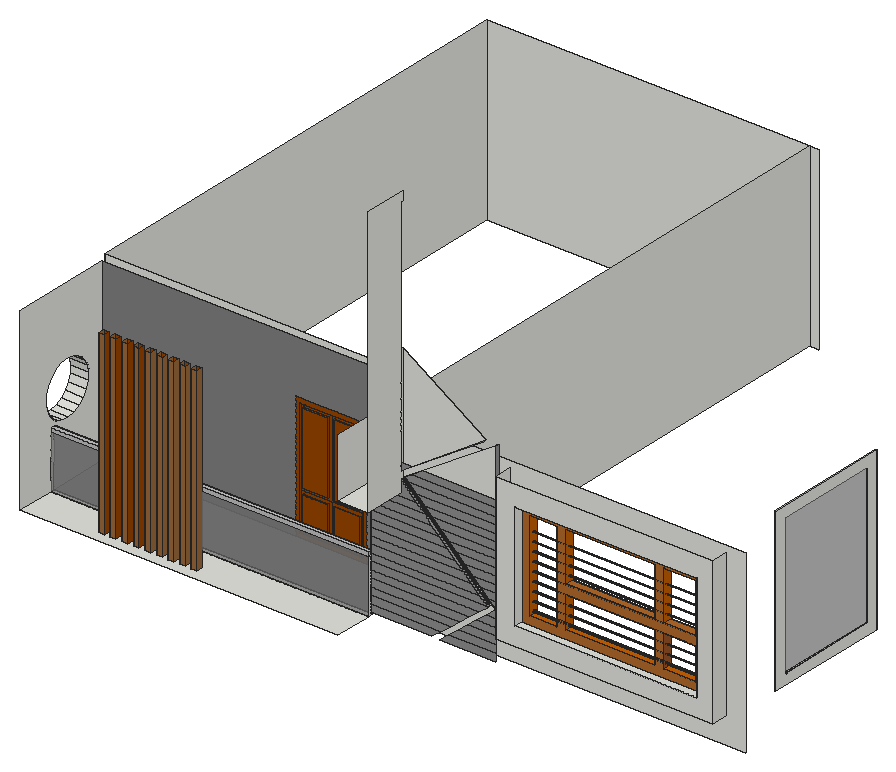
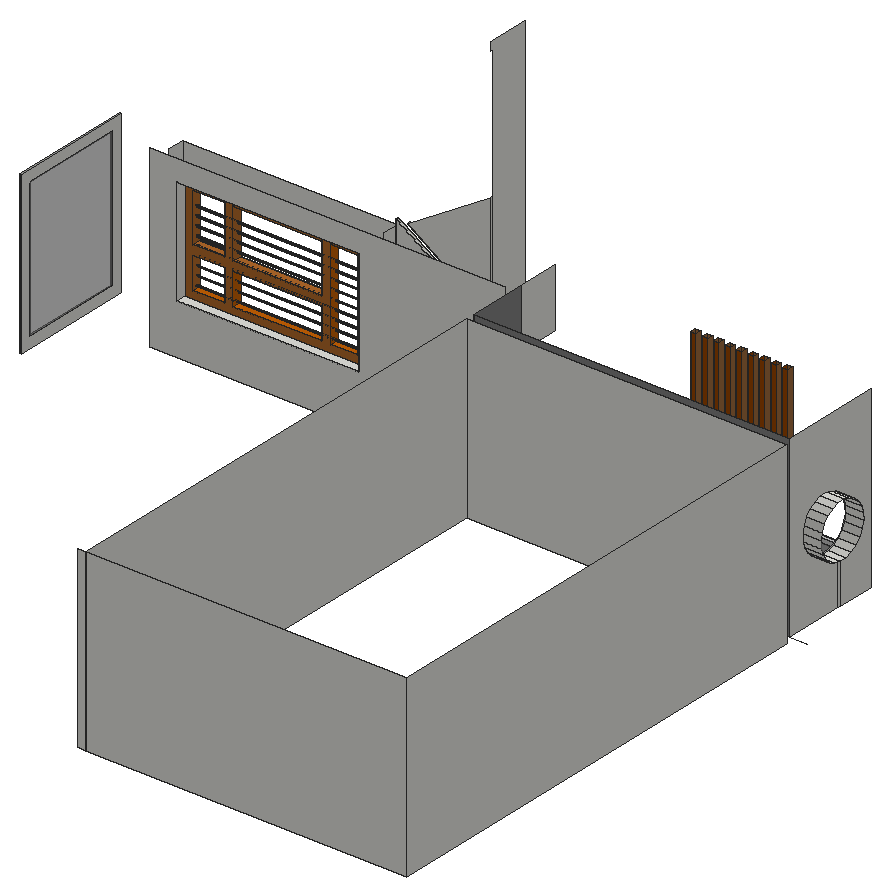
# SketchUp Ruby script. Lengths in inches.
U = 1.inch
M = Sketchup.active_model
def pt(a) = Geom::Point3d.new(a.map { |v| v * U })
def face(e, loops, mat)
  f = e.add_face(loops[0].map { |a| pt(a) })
  loops[1..].each { |l| e.add_face(l.map { |a| pt(a) }).erase! }
  f.material = f.back_material = mat if mat
  f
end
# faces: each face lists its corners as indices into pts; further lists are holes
def faces(e, pts, list, mat = nil) = list.each { |f| face(e, (f[0].is_a?(Array) ? f : [f]).map { |l| l.map { |i| pts[i] } }, mat) }
# xy, xz, yz: faces in a plane at the given z, y or x. An outline is a flat list of corners, or four numbers for a rectangle; further outlines are holes
def ring(l) = l.size == 4 ? [[l[0], l[1]], [l[2], l[1]], [l[2], l[3]], [l[0], l[3]]] : l.each_slice(2).to_a
def flat(e, list, mat, &to3) = list.each { |f| face(e, (f[0].is_a?(Array) ? f : [f]).map { |l| ring(l).map { |u, v| to3.(u, v) } }, mat) }
def xy(e, z, list, mat = nil) = flat(e, list, mat) { |x, y| [x, y, z] }
def xz(e, y, list, mat = nil) = flat(e, list, mat) { |x, z| [x, y, z] }
def yz(e, x, list, mat = nil) = flat(e, list, mat) { |y, z| [x, y, z] }
def lines(e, pts, list) = list.each { |a, b| e.add_line(pt(pts[a]), pt(pts[b])) }
# prism: a flat outline (further loops are holes) pulled along v
def prism(e, loops, v, mat = nil)
  f = face(e, loops, mat); d = Geom::Vector3d.new(v.map { |x| x * U })
  f.pushpull(f.normal.samedirection?(d) ? d.length : -d.length)
end
def box(e, o, s, mat = nil) = prism(e, [[o, [o[0] + s[0], o[1], o[2]], [o[0] + s[0], o[1] + s[1], o[2]], [o[0], o[1] + s[1], o[2]]]], [0, 0, s[2]], mat)
def at(x, y, z, deg = 0) = Geom::Transformation.translation(pt([x, y, z])) * Geom::Transformation.rotation(ORIGIN, Z_AXIS, deg.degrees)
def axes(o, x, y, z) = Geom::Transformation.new([*x, 0, *y, 0, *z, 0, *pt(o).to_a, 1])
def part(name) = M.definitions.add(name)
# library, detail: a bought-in or finely detailed component or shape, given as its bounding box
def library(name, o, s) = part(name).tap { |d| box(d.entities, o, s) }
def detail(e, o, s) = box(e.add_group.entities, o, s)
def put(e, d, t, mat = nil) = e.add_instance(d, t).tap { |i| i.material = mat if mat }
def group(e, t, mat = nil) = e.add_group.tap { |g| g.transformation = t; g.material = mat if mat }.entities
root = M.entities
M.materials.add("[0132_LightGray]").color = [169, 169, 169]
M.materials.add("[0133_Gray]").color = [128, 128, 128]
M.materials.add("[Color M04]").color = [142, 142, 142]
M.materials.add("[Metal Corrugated Shiny]").color = [193, 193, 193]
M.materials.add("[Stone Vein Gray]").color = [166, 165, 165]
M.materials.add("[Translucent Glass Gray]").color = [128, 128, 128]
M.materials["[Translucent Glass Gray]"].alpha = 0.68
M.materials.add("[Wood Bamboo]").color = [195, 96, 5]
M.materials.add("[Wood Bamboo]1").color = [177, 105, 43]
M.materials.add("[Wood Cherry Original]").color = [152, 68, 0]
M.materials.add("[Wood Cherry Original]1").color = [152, 86, 42]
M.materials.add("[Wood Floor]").color = [155, 105, 61]
xy(root,218,[[[28.03,15.6875,241.25,41],[74.77,23.01,78.7,26.95],[82.52,23.01,86.45,26.95],[90.27,23.01,94.2,26.95],[98.02,23.01,101.95,26.95],[105.77,23.01,109.7,26.95],[113.52,23.01,117.45,26.95],[121.27,23.01,125.2,26.95],[129.02,23.01,132.95,26.95],[136.77,23.01,140.7,26.95]],[28.03,41,241.25,44]])
xy(root,218,[[28.03,44,241.25,84.25]],"[Stone Vein Gray]")
xy(root,218,[[74.77,23.01,78.7,26.95],[82.52,23.01,86.45,26.95],[90.27,23.01,94.2,26.95],[98.02,23.01,101.95,26.95],[105.77,23.01,109.7,26.95],
  [113.52,23.01,117.45,26.95],[121.27,23.01,125.2,26.95],[129.02,23.01,132.95,26.95],[136.77,23.01,140.7,26.95]],"[Wood Cherry Original]")
xy(root,220.79,[[160.66,84.25,203.09,84.75]],"[Wood Cherry Original]")
xy(root,222.79,[[162.66,83.75,179.875,84.75]])
xy(root,222.82,[[183.91,83.75,201.05,84.75]])
xy(root,239.94,[[333.13,33.25,478.31,44.6875]])
xy(root,244.7,[[183.91,83.75,201.05,84.75]],"[Wood Cherry Original]")
xy(root,244.74,[[162.66,83.75,179.875,84.75]],"[Wood Cherry Original]")
xy(root,248.74,[[162.66,83.75,179.875,84.75],[183.875,83.75,201.09,84.75]])
xy(root,252.35,[[345.84,33.25,468.09,38.65],[345.84,44.67,468.09,50.6875]])
xy(root,253,[[495.875,63.375,496.875,147.375]])
xy(root,254,[[28.03,41,241.25,44]],"[Metal Corrugated Shiny]")
xy(root,256.625,[[28.03,41,241.25,44]],"[Metal Corrugated Shiny]")
xy(root,257.74,[[351.24,38.65,369.24,44.67],[375.24,38.65,435.1,44.67],[441.1,38.65,462.7,44.67]],"[Wood Bamboo]")
xy(root,260,[[495.875,70.375,496.875,140.375]])
xy(root,279.34,[[375.24,38.65,435.1,44.67],[441.1,38.65,462.7,44.67]])
xy(root,285.34,[[375.24,38.65,435.1,44.67],[441.1,38.65,462.7,44.67]],"[Wood Bamboo]1")
xy(root,297.21,[[162.66,83.75,179.875,84.75],[183.875,83.75,201.09,84.75]],"[Wood Cherry Original]")
xy(root,298.5,[[241.25,15.6875,261.37,42.75],[241.25,42.75,261.37,44.4375],[241.25,44.4375,261.37,44.6875]])
xy(root,299.21,[[160.66,84.25,203.09,84.75]])
xz(root,23.01,[[74.77,218,78.7,338],[82.52,218,86.45,338],[90.27,218,94.2,338],[98.02,218,101.95,338],[105.77,218,109.7,338],
  [113.52,218,117.45,338],[121.27,218,125.2,338],[129.02,218,132.95,338],[136.77,218,140.7,338]],"[Wood Floor]")
xz(root,26.95,[[74.77,218,78.7,338],[82.52,218,86.45,338],[90.27,218,94.2,338],[98.02,218,101.95,338],[105.77,218,109.7,338],
  [113.52,218,117.45,338],[121.27,218,125.2,338],[129.02,218,132.95,338],[136.77,218,140.7,338]],"[Wood Cherry Original]")
xz(root,33.25,[[[333.13,239.94,478.31,337.75],[345.84,252.35,468.09,323.97]]])
xz(root,38.65,[[[345.84,252.35,468.09,323.97],[375.24,257.74,375.24,279.34,435.1,279.34,435.1,257.74,441.1,257.74,441.1,279.34,462.7,279.34,462.7,285.34,441.1,285.34,441.1,318.58,462.7,318.58,462.7,257.74],[375.24,285.34,435.1,318.58],[351.24,257.74,369.24,318.58]]],"[Wood Bamboo]1")
xz(root,41,[[28.03,254,241.25,256.625]],"[Metal Corrugated Shiny]")
xz(root,41,[[28.03,218,241.25,254]],"[Translucent Glass Gray]")
xz(root,42.75,[[325.43,250.42,325.49,250.42,325.49,250.46]])
xz(root,42.75,[[241.25,219.67,282.3,219.67,288.6,224.79,241.25,224.79],[287.88,219.67,325.49,219.67,325.49,224.79,294.14,224.79],[241.25,224.79,288.6,224.79,294.9,229.92,241.25,229.92],[294.14,224.79,325.49,224.79,325.49,229.92,300.4,229.92],[241.25,229.92,294.9,229.92,301.2,235.04,241.25,235.04],
  [300.4,229.92,325.49,229.92,325.49,235.04,306.66,235.04],[241.25,235.04,301.2,235.04,307.51,240.17,241.25,240.17],[306.66,235.04,325.49,235.04,325.49,240.17,312.92,240.17],[241.25,240.17,307.51,240.17,313.81,245.29,241.25,245.29],[312.92,240.17,325.49,240.17,325.49,245.29,319.17,245.29],
  [241.25,245.29,313.81,245.29,319.9,250.25,319.73,250.42,241.25,250.42],[319.17,245.29,325.49,245.29,325.49,250.42,325.43,250.42],[241.25,250.42,319.73,250.42,314.4375,255.54,241.25,255.54],[325.49,250.46,325.49,255.54,320.17,255.54],[241.25,255.54,314.4375,255.54,309.15,260.67,241.25,260.67],
  [320.17,255.54,325.49,255.54,325.49,260.67,314.8125,260.67],[241.25,260.67,309.15,260.67,303.86,265.79,241.25,265.79],[314.8125,260.67,325.49,260.67,325.49,265.79,309.45,265.79],[241.25,265.79,303.86,265.79,298.57,270.92,241.25,270.92],[309.45,265.79,325.49,265.79,325.49,270.92,304.09,270.92],
  [241.25,270.92,298.57,270.92,293.28,276.04,241.25,276.04],[304.09,270.92,325.49,270.92,325.49,276.04,298.73,276.04],[241.25,276.04,293.28,276.04,287.99,281.17,241.25,281.17],[298.73,276.04,325.49,276.04,325.49,281.17,293.375,281.17],[241.25,281.17,287.99,281.17,282.7,286.29,241.25,286.29],
  [293.375,281.17,325.49,281.17,325.49,286.29,288.01,286.29],[241.25,286.29,282.7,286.29,277.41,291.42,241.25,291.42],[288.01,286.29,325.49,286.29,325.49,291.42,282.65,291.42],[241.25,291.42,277.41,291.42,272.125,296.54,241.25,296.54],[282.65,291.42,325.49,291.42,325.49,296.54,277.3,296.54],
  [241.25,296.54,272.125,296.54,261.37,306.96,261.37,298.5,241.25,298.5],[277.3,296.54,325.49,296.54,325.49,301.67,271.9375,301.67],[271.9375,301.67,325.49,301.67,325.49,306.79,266.58,306.79],[266.58,306.79,325.49,306.79,325.49,311.92,268.9,311.92,264.35,308.92],[261.37,311.77,269.28,317.04,261.37,317.04],
  [268.9,311.92,325.49,311.92,325.49,317.04,276.6875,317.04]],"[Color M04]")
xz(root,44,[[28.03,254,241.25,256.625]],"[Metal Corrugated Shiny]")
xz(root,44,[[28.03,218,241.25,254]],"[Translucent Glass Gray]")
xz(root,44.67,[[[345.84,252.35,468.09,323.97],[375.24,285.34,435.1,318.58],[375.24,257.74,435.1,279.34],[351.24,257.74,369.24,318.58],[441.1,285.34,462.7,318.58],[441.1,257.74,462.7,279.34]]],"[Wood Bamboo]1")
xz(root,44.6875,[[325.49,250.46,264.35,308.92,325.49,349.15],[261.37,311.77,261.37,384.6,317.38,349.1]])
xz(root,50.6875,[[[247.25,218,486.875,338],[345.84,252.35,468.09,323.97]]])
xz(root,63.375,[[495.875,253,496.875,361]])
xz(root,70.375,[[495.875,260,496.875,354]])
xz(root,83.75,[[162.66,222.79,179.875,244.74],[183.91,222.82,201.05,244.7],[162.66,248.74,179.875,297.21],[183.875,248.74,201.09,297.21]],"[Wood Cherry Original]")
xz(root,84.25,[[28.03,218,157.875,218,157.875,302,205.875,302,205.875,218,241.25,218,241.25,338,28.03,338]],"[0133_Gray]")
xz(root,84.25,[[[157.875,218,205.875,302],[160.66,220.79,203.09,299.21]]],"[Wood Cherry Original]")
xz(root,84.75,[[[160.66,220.79,181.875,246.74],[162.66,222.79,179.875,244.74]],[[181.875,220.79,203.09,246.74],[183.91,222.82,201.05,244.7]],[[160.66,246.74,181.875,299.21],[162.66,248.74,179.875,297.21]],[[181.875,246.74,203.09,299.21],[183.875,248.74,201.09,297.21]]],"[Wood Cherry Original]")
xz(root,90.25,[[24.875,218,241.25,338]])
xz(root,140.375,[[495.875,260,496.875,354]])
xz(root,147.375,[[495.875,253,496.875,361]])
xz(root,411,[[24.875,218,241.25,338],[241.25,218,247.25,338]])
yz(root,24.875,[[90.25,218,411,338]])
yz(root,28.03,[[[15.6875,218,41,218,41,256.625,44,256.625,44,218,84.25,218,84.25,338,15.6875,338],[56.56,256.125,51.83,256.36,47.33,257.82,43.36,260.38,40.19,263.89,38.03,268.11,37.04,272.73,37.27,277.46,38.73,281.96,41.3,285.93,44.81,289.11,49.02,291.26,53.64,292.26,58.37,292.02,62.87,290.57,66.85,288,70.02,284.49,72.18,280.27,73.17,275.65,72.93,270.92,71.48,266.42,68.91,262.45,65.4,259.27,61.1875,257.12]],[41,218,44,254]])
yz(root,28.03,[[41,254,44,256.625]],"[Metal Corrugated Shiny]")
yz(root,74.77,[[23.01,218,26.95,338]],"[Wood Floor]")
yz(root,78.7,[[23.01,218,26.95,338]],"[Wood Cherry Original]")
yz(root,82.52,[[23.01,218,26.95,338]],"[Wood Floor]")
yz(root,86.45,[[23.01,218,26.95,338]],"[Wood Cherry Original]")
yz(root,90.27,[[23.01,218,26.95,338]],"[Wood Floor]")
yz(root,94.2,[[23.01,218,26.95,338]],"[Wood Cherry Original]")
yz(root,98.02,[[23.01,218,26.95,338]],"[Wood Floor]")
yz(root,101.95,[[23.01,218,26.95,338]],"[Wood Cherry Original]")
yz(root,105.77,[[23.01,218,26.95,338]],"[Wood Floor]")
yz(root,109.7,[[23.01,218,26.95,338]],"[Wood Floor]")
yz(root,113.52,[[23.01,218,26.95,338]],"[Wood Floor]")
yz(root,117.45,[[23.01,218,26.95,338]],"[Wood Floor]")
yz(root,121.27,[[23.01,218,26.95,338]],"[Wood Floor]")
yz(root,125.2,[[23.01,218,26.95,338]],"[Wood Floor]")
yz(root,129.02,[[23.01,218,26.95,338]],"[Wood Floor]")
yz(root,132.95,[[23.01,218,26.95,338]],"[Wood Floor]")
yz(root,136.77,[[23.01,218,26.95,338]],"[Wood Floor]")
yz(root,140.7,[[23.01,218,26.95,338]],"[Wood Floor]")
yz(root,160.66,[[84.25,220.79,84.75,299.21]],"[Wood Cherry Original]")
yz(root,162.66,[[83.75,222.79,84.75,244.74]])
yz(root,162.66,[[83.75,248.74,84.75,297.21]],"[Wood Cherry Original]")
yz(root,179.875,[[83.75,222.79,84.75,244.74],[83.75,248.74,84.75,297.21]],"[Wood Cherry Original]")
yz(root,183.875,[[83.75,248.74,84.75,297.21]],"[Wood Cherry Original]")
yz(root,183.91,[[83.75,222.82,84.75,244.7]],"[Wood Cherry Original]")
yz(root,201.05,[[83.75,222.82,84.75,244.7]],"[Wood Cherry Original]")
yz(root,201.09,[[83.75,248.74,84.75,297.21]],"[Wood Cherry Original]")
yz(root,203.09,[[84.25,220.79,84.75,299.21]],"[Wood Cherry Original]")
yz(root,241.25,[[41,218,42.75,254],[42.75,218,44,254],[44,218,44,256.625,42.75,256.625,42.75,298.5,44.4375,298.5,44.4375,218],[44.4375,218,44.6875,298.5],[90.25,218,411,338],
  [15.6875,298.5,44.6875,338]])
yz(root,241.25,[[44.6875,218,84.25,338]],"[0133_Gray]")
yz(root,241.25,[[41,254,42.75,256.625],[42.75,254,44,256.625]],"[Metal Corrugated Shiny]")
yz(root,261.37,[[15.6875,298.5,42.75,298.5,42.75,306.96,44.6875,306.96,44.6875,311.77,42.75,311.77,42.75,473.32,44.6875,473.32,44.6875,479,15.6875,479],[42.75,298.5,44.4375,306.96],[44.4375,298.5,44.6875,306.96],[42.75,311.77,44.6875,384.6]])
yz(root,325.49,[[42.75,250.46,44.6875,349.15]],"[Color M04]")
yz(root,333.13,[[33.25,239.94,44.6875,337.75]])
yz(root,345.84,[[33.25,252.35,38.65,323.97],[44.67,252.35,50.6875,323.97]])
yz(root,351.24,[[38.65,257.74,41.66,257.74,41.66,259.01,41.53,259.02,41.41,259.07,41.31,259.15,41.23,259.26,41.18,259.375,41.16,259.51,41.18,259.63,41.23,259.76,41.31,259.86,41.41,259.9375,41.53,259.99,41.66,260.01,41.79,259.99,41.91,259.9375,42.01,259.86,42.09,259.76,42.14,259.63,42.16,259.51,42.14,259.375,42.09,259.26,42.01,259.15,41.91,259.07,41.79,259.02,41.66,259.01,41.66,257.74,44.67,257.74,44.67,318.58,38.65,318.58]],"[Wood Bamboo]")
yz(root,369.24,[[38.65,257.74,44.67,318.58]],"[Wood Bamboo]")
yz(root,375.24,[[38.65,257.74,44.67,279.34],[38.65,285.34,44.67,318.58]],"[Wood Bamboo]")
yz(root,435.1,[[38.65,257.74,44.67,279.34]],"[Wood Bamboo]")
yz(root,435.1,[[38.65,285.34,44.67,318.58]],"[Wood Bamboo]1")
yz(root,441.1,[[38.65,285.34,44.67,318.58]],"[Wood Bamboo]")
yz(root,441.1,[[38.65,257.74,44.67,279.34]],"[Wood Cherry Original]1")
yz(root,462.7,[[[38.65,257.74,44.67,279.34],[41.66,259.01,41.79,259.02,41.91,259.07,42.01,259.15,42.09,259.26,42.14,259.375,42.16,259.51,42.14,259.63,42.09,259.76,42.01,259.86,41.91,259.9375,41.79,259.99,41.66,260.01,41.53,259.99,41.41,259.9375,41.31,259.86,41.23,259.76,41.18,259.63,41.16,259.51,41.18,259.375,41.23,259.26,41.31,259.15,41.41,259.07,41.53,259.02]],[38.65,285.34,44.67,318.58]],"[Wood Bamboo]1")
yz(root,468.09,[[33.25,252.35,38.65,323.97],[44.67,252.35,50.6875,323.97]])
yz(root,478.31,[[33.25,239.94,44.6875,337.75]])
yz(root,495.875,[[[63.375,253,147.375,361],[70.375,260,140.375,354]]])
yz(root,495.875,[[70.375,260,140.375,354]],"[Translucent Glass Gray]")
yz(root,496.875,[[[63.375,253,147.375,361],[70.375,260,140.375,354]]])
p = [[261.37,42.75,306.96],[272.125,42.75,296.54],[277.41,42.75,291.42],[282.7,42.75,286.29],[287.99,42.75,281.17],[293.28,42.75,276.04],
  [298.57,42.75,270.92],[303.86,42.75,265.79],[309.15,42.75,260.67],[314.4375,42.75,255.54],[319.73,42.75,250.42],[319.9,42.75,250.25],
  [319.9,44.4375,250.25],[261.37,44.4375,306.96],[319.9,44.6875,250.25],[261.37,44.6875,306.96],[264.35,44.6875,308.92],[325.49,44.6875,250.46],
  [325.49,42.75,250.46],[320.17,42.75,255.54],[314.8125,42.75,260.67],[309.45,42.75,265.79],[304.09,42.75,270.92],[298.73,42.75,276.04],
  [293.375,42.75,281.17],[288.01,42.75,286.29],[282.65,42.75,291.42],[277.3,42.75,296.54],[271.9375,42.75,301.67],[266.58,42.75,306.79],
  [264.35,42.75,308.92],[28.03,51.83,256.36],[28.03,56.56,256.125],[15.875,56.56,256.125],[15.875,51.83,256.36],[28.03,61.1875,257.12],
  [15.875,61.1875,257.12],[28.03,47.33,257.82],[15.875,47.33,257.82],[28.03,65.4,259.27],[15.875,65.4,259.27],[28.03,43.36,260.38],
  [15.875,43.36,260.38],[351.24,41.41,259.07],[351.24,41.53,259.02],[462.7,41.53,259.02],[462.7,41.41,259.07],[351.24,41.66,259.01],
  [462.7,41.66,259.01],[351.24,41.79,259.02],[462.7,41.79,259.02],[351.24,41.91,259.07],[462.7,41.91,259.07],[351.24,41.31,259.15],
  [462.7,41.31,259.15],[351.24,42.01,259.15],[462.7,42.01,259.15],[351.24,41.23,259.26],[462.7,41.23,259.26],[351.24,42.09,259.26],
  [462.7,42.09,259.26],[351.24,41.18,259.375],[462.7,41.18,259.375],[351.24,42.14,259.375],[462.7,42.14,259.375],[28.03,68.91,262.45],
  [15.875,68.91,262.45],[351.24,41.16,259.51],[462.7,41.16,259.51],[351.24,42.16,259.51],[462.7,42.16,259.51],[351.24,41.18,259.63],
  [462.7,41.18,259.63],[351.24,42.14,259.63],[462.7,42.14,259.63],[351.24,41.23,259.76],[462.7,41.23,259.76],[351.24,42.09,259.76],
  [462.7,42.09,259.76],[351.24,41.31,259.86],[462.7,41.31,259.86],[351.24,42.01,259.86],[462.7,42.01,259.86],[351.24,41.41,259.9375],
  [462.7,41.41,259.9375],[351.24,41.53,259.99],[462.7,41.53,259.99],[351.24,41.91,259.9375],[351.24,41.79,259.99],[462.7,41.79,259.99],
  [462.7,41.91,259.9375],[351.24,41.66,260.01],[462.7,41.66,260.01],[28.03,40.19,263.89],[15.875,40.19,263.89],[28.03,71.48,266.42],
  [15.875,71.48,266.42],[28.03,38.03,268.11],[15.875,38.03,268.11],[351.24,41.41,265.07],[351.24,41.53,265.02],[462.7,41.53,265.02],
  [462.7,41.41,265.07],[351.24,41.66,265.01],[462.7,41.66,265.01],[351.24,41.31,265.15],[462.7,41.31,265.15],[351.24,41.23,265.26],
  [462.7,41.23,265.26],[351.24,41.18,265.375],[462.7,41.18,265.375],[351.24,41.16,265.51],[462.7,41.16,265.51],[351.24,41.18,265.63],
  [462.7,41.18,265.63],[351.24,41.23,265.76],[462.7,41.23,265.76],[351.24,41.31,265.86],[462.7,41.31,265.86],[351.24,41.41,265.9375],
  [462.7,41.41,265.9375],[351.24,41.53,265.99],[462.7,41.53,265.99],[351.24,41.66,266.01],[462.7,41.66,266.01],[28.03,72.93,270.92],
  [15.875,72.93,270.92],[28.03,37.04,272.73],[15.875,37.04,272.73],[28.03,73.17,275.65],[15.875,73.17,275.65],[351.24,41.41,271.07],
  [351.24,41.53,271.02],[462.7,41.53,271.02],[462.7,41.41,271.07],[351.24,41.66,271.01],[462.7,41.66,271.01],[351.24,41.31,271.15],
  [462.7,41.31,271.15],[351.24,41.23,271.26],[462.7,41.23,271.26],[351.24,41.18,271.375],[462.7,41.18,271.375],[351.24,41.16,271.51],
  [462.7,41.16,271.51],[351.24,41.18,271.63],[462.7,41.18,271.63],[351.24,41.23,271.76],[462.7,41.23,271.76],[351.24,41.31,271.86],
  [462.7,41.31,271.86],[351.24,41.41,271.9375],[462.7,41.41,271.9375],[351.24,41.53,271.99],[462.7,41.53,271.99],[351.24,41.66,272.01],
  [462.7,41.66,272.01],[28.03,37.27,277.46],[15.875,37.27,277.46],[28.03,72.18,280.27],[15.875,72.18,280.27],[351.24,41.41,277.07],
  [351.24,41.53,277.02],[462.7,41.53,277.02],[462.7,41.41,277.07],[351.24,41.66,277.01],[462.7,41.66,277.01],[351.24,41.31,277.15],
  [462.7,41.31,277.15],[351.24,41.23,277.26],[462.7,41.23,277.26],[351.24,41.18,277.375],[462.7,41.18,277.375],[351.24,41.16,277.51],
  [462.7,41.16,277.51],[28.03,38.73,281.96],[15.875,38.73,281.96],[351.24,41.18,277.63],[462.7,41.18,277.63],[351.24,41.23,277.76],
  [462.7,41.23,277.76],[351.24,41.31,277.86],[462.7,41.31,277.86],[351.24,41.41,277.9375],[462.7,41.41,277.9375],[351.24,41.53,277.99],
  [462.7,41.53,277.99],[351.24,41.66,278.01],[462.7,41.66,278.01],[28.03,70.02,284.49],[15.875,70.02,284.49],[28.03,41.3,285.93],
  [15.875,41.3,285.93],[351.24,41.41,283.07],[351.24,41.53,283.02],[462.7,41.53,283.02],[462.7,41.41,283.07],[351.24,41.66,283.01],
  [462.7,41.66,283.01],[351.24,41.31,283.15],[462.7,41.31,283.15],[351.24,41.23,283.26],[462.7,41.23,283.26],[351.24,41.18,283.375],
  [462.7,41.18,283.375],[351.24,41.16,283.51],[462.7,41.16,283.51],[351.24,41.18,283.63],[462.7,41.18,283.63],[351.24,41.23,283.76],
  [462.7,41.23,283.76],[351.24,41.31,283.86],[462.7,41.31,283.86],[351.24,41.41,283.9375],[462.7,41.41,283.9375],[351.24,41.53,283.99],
  [462.7,41.53,283.99],[351.24,41.66,284.01],[462.7,41.66,284.01],[28.03,66.85,288],[15.875,66.85,288],[28.03,44.81,289.11],
  [15.875,44.81,289.11],[28.03,62.87,290.57],[15.875,62.87,290.57],[351.24,41.41,289.07],[351.24,41.53,289.02],[462.7,41.53,289.02],
  [462.7,41.41,289.07],[351.24,41.66,289.01],[462.7,41.66,289.01],[351.24,41.31,289.15],[462.7,41.31,289.15],[28.03,49.02,291.26],
  [15.875,49.02,291.26],[351.24,41.23,289.26],[462.7,41.23,289.26],[351.24,41.18,289.375],[462.7,41.18,289.375],[351.24,41.16,289.51],
  [462.7,41.16,289.51],[351.24,41.18,289.63],[462.7,41.18,289.63],[351.24,41.23,289.76],[462.7,41.23,289.76],[351.24,41.31,289.86],
  [462.7,41.31,289.86],[351.24,41.41,289.9375],[462.7,41.41,289.9375],[351.24,41.53,289.99],[462.7,41.53,289.99],[351.24,41.66,290.01],
  [462.7,41.66,290.01],[28.03,58.37,292.02],[15.875,58.37,292.02],[28.03,53.64,292.26],[15.875,53.64,292.26],[351.24,41.41,295.07],
  [351.24,41.53,295.02],[462.7,41.53,295.02],[462.7,41.41,295.07],[351.24,41.66,295.01],[462.7,41.66,295.01],[351.24,41.31,295.15],
  [462.7,41.31,295.15],[351.24,41.23,295.26],[462.7,41.23,295.26],[351.24,41.18,295.375],[462.7,41.18,295.375],[351.24,41.16,295.51],
  [462.7,41.16,295.51],[351.24,41.18,295.63],[462.7,41.18,295.63],[351.24,41.23,295.76],[462.7,41.23,295.76],[351.24,41.31,295.86],
  [462.7,41.31,295.86],[351.24,41.41,295.9375],[462.7,41.41,295.9375],[351.24,41.53,295.99],[462.7,41.53,295.99],[351.24,41.66,296.01],
  [462.7,41.66,296.01],[351.24,41.41,301.07],[351.24,41.53,301.02],[462.7,41.53,301.02],[462.7,41.41,301.07],[351.24,41.66,301.01],
  [462.7,41.66,301.01],[351.24,41.31,301.15],[462.7,41.31,301.15],[351.24,41.23,301.26],[462.7,41.23,301.26],[351.24,41.18,301.375],
  [462.7,41.18,301.375],[351.24,41.16,301.51],[462.7,41.16,301.51],[351.24,41.18,301.63],[462.7,41.18,301.63],[351.24,41.23,301.76],
  [462.7,41.23,301.76],[351.24,41.31,301.86],[462.7,41.31,301.86],[351.24,41.41,301.9375],[462.7,41.41,301.9375],[351.24,41.53,301.99],
  [462.7,41.53,301.99],[351.24,41.66,302.01],[462.7,41.66,302.01],[351.24,41.41,307.07],[351.24,41.53,307.02],[462.7,41.53,307.02],
  [462.7,41.41,307.07],[351.24,41.66,307.01],[462.7,41.66,307.01],[351.24,41.31,307.15],[462.7,41.31,307.15],[351.24,41.23,307.26],
  [462.7,41.23,307.26],[351.24,41.18,307.375],[462.7,41.18,307.375],[351.24,41.16,307.51],[462.7,41.16,307.51],[351.24,41.18,307.63],
  [462.7,41.18,307.63],[351.24,41.23,307.76],[462.7,41.23,307.76],[351.24,41.31,307.86],[462.7,41.31,307.86],[351.24,41.41,307.9375],
  [462.7,41.41,307.9375],[351.24,41.53,307.99],[462.7,41.53,307.99],[351.24,41.66,308.01],[462.7,41.66,308.01],[325.49,44.6875,349.15],
  [268.9,42.75,311.92],[276.6875,42.75,317.04],[284.48,42.75,322.17],[292.26,42.75,327.29],[300.05,42.75,332.42],[307.84,42.75,337.54],
  [315.63,42.75,342.67],[323.42,42.75,347.79],[325.49,42.75,349.15],[261.37,44.6875,311.77],[317.38,44.6875,349.1],[317.38,42.75,349.1],
  [315.42,42.75,347.79],[307.73,42.75,342.67],[300.04,42.75,337.54],[292.35,42.75,332.42],[284.66,42.75,327.29],[276.97,42.75,322.17],
  [269.28,42.75,317.04],[261.37,42.75,311.77],[15.875,84.25,218],[28.03,84.25,218]]
faces(root,p,[[0,1,2,3,4,5,6,7,8,9,10,11,12,13],[16,17,18,19,20,21,22,23,24,25,26,27,28,29,30],[345,346,347,348,349,350,351,352,353,354,355]],"[Color M04]")
faces(root,p,[[14,15,13,12],[31,32,33,34],[32,35,36,33],[37,31,34,38],[35,39,40,36],[41,37,38,42],[47,49,50,48],[49,51,52,50],
  [51,55,56,52],[55,59,60,56],[59,63,64,60],[39,65,66,40],[63,69,70,64],[69,73,74,70],[73,77,78,74],[77,81,82,78],
  [87,88,89,90],[81,87,90,82],[88,91,92,89],[93,41,42,94],[65,95,96,66],[97,93,94,98],[95,125,126,96],[127,97,98,128],
  [125,129,130,126],[157,127,128,158],[129,159,160,130],[175,157,158,176],[159,189,190,160],[191,175,176,192],[189,219,220,190],[221,191,192,222],
  [219,223,224,220],[233,221,222,234],[223,253,254,224],[255,233,234,256],[253,255,256,254],[335,16,30,336,337,338,339,340,341,342,343,344]])
faces(root,p,[[43,44,45,46],[44,47,48,45],[53,43,46,54],[57,53,54,58],[61,57,58,62],[67,61,62,68],[71,67,68,72],[75,71,72,76],
  [79,75,76,80],[83,79,80,84],[85,83,84,86],[91,85,86,92],[99,100,101,102],[100,103,104,101],[105,99,102,106],[107,105,106,108],
  [109,107,108,110],[111,109,110,112],[113,111,112,114],[115,113,114,116],[117,115,116,118],[119,117,118,120],[121,119,120,122],[123,121,122,124],
  [131,132,133,134],[132,135,136,133],[137,131,134,138],[139,137,138,140],[141,139,140,142],[143,141,142,144],[145,143,144,146],[147,145,146,148],
  [149,147,148,150],[151,149,150,152],[153,151,152,154],[155,153,154,156],[161,162,163,164],[162,165,166,163],[167,161,164,168],[169,167,168,170],
  [171,169,170,172],[173,171,172,174],[177,173,174,178],[179,177,178,180],[181,179,180,182],[183,181,182,184],[185,183,184,186],[187,185,186,188],
  [193,194,195,196],[194,197,198,195],[199,193,196,200],[201,199,200,202],[203,201,202,204],[205,203,204,206],[207,205,206,208],[209,207,208,210],
  [211,209,210,212],[213,211,212,214],[215,213,214,216],[217,215,216,218],[225,226,227,228],[226,229,230,227],[231,225,228,232],[235,231,232,236],
  [237,235,236,238],[239,237,238,240],[241,239,240,242],[243,241,242,244],[245,243,244,246],[247,245,246,248],[249,247,248,250],[251,249,250,252],
  [257,258,259,260],[258,261,262,259],[263,257,260,264],[265,263,264,266],[267,265,266,268],[269,267,268,270],[271,269,270,272],[273,271,272,274],
  [275,273,274,276],[277,275,276,278],[279,277,278,280],[281,279,280,282],[283,284,285,286],[284,287,288,285],[289,283,286,290],[291,289,290,292],
  [293,291,292,294],[295,293,294,296],[297,295,296,298],[299,297,298,300],[301,299,300,302],[303,301,302,304],[305,303,304,306],[307,305,306,308],
  [309,310,311,312],[310,313,314,311],[315,309,312,316],[317,315,316,318],[319,317,318,320],[321,319,320,322],[323,321,322,324],[325,323,324,326],
  [327,325,326,328],[329,327,328,330],[331,329,330,332],[333,331,332,334]],"[0132_LightGray]")
lines(root,p,[[356,357]])
